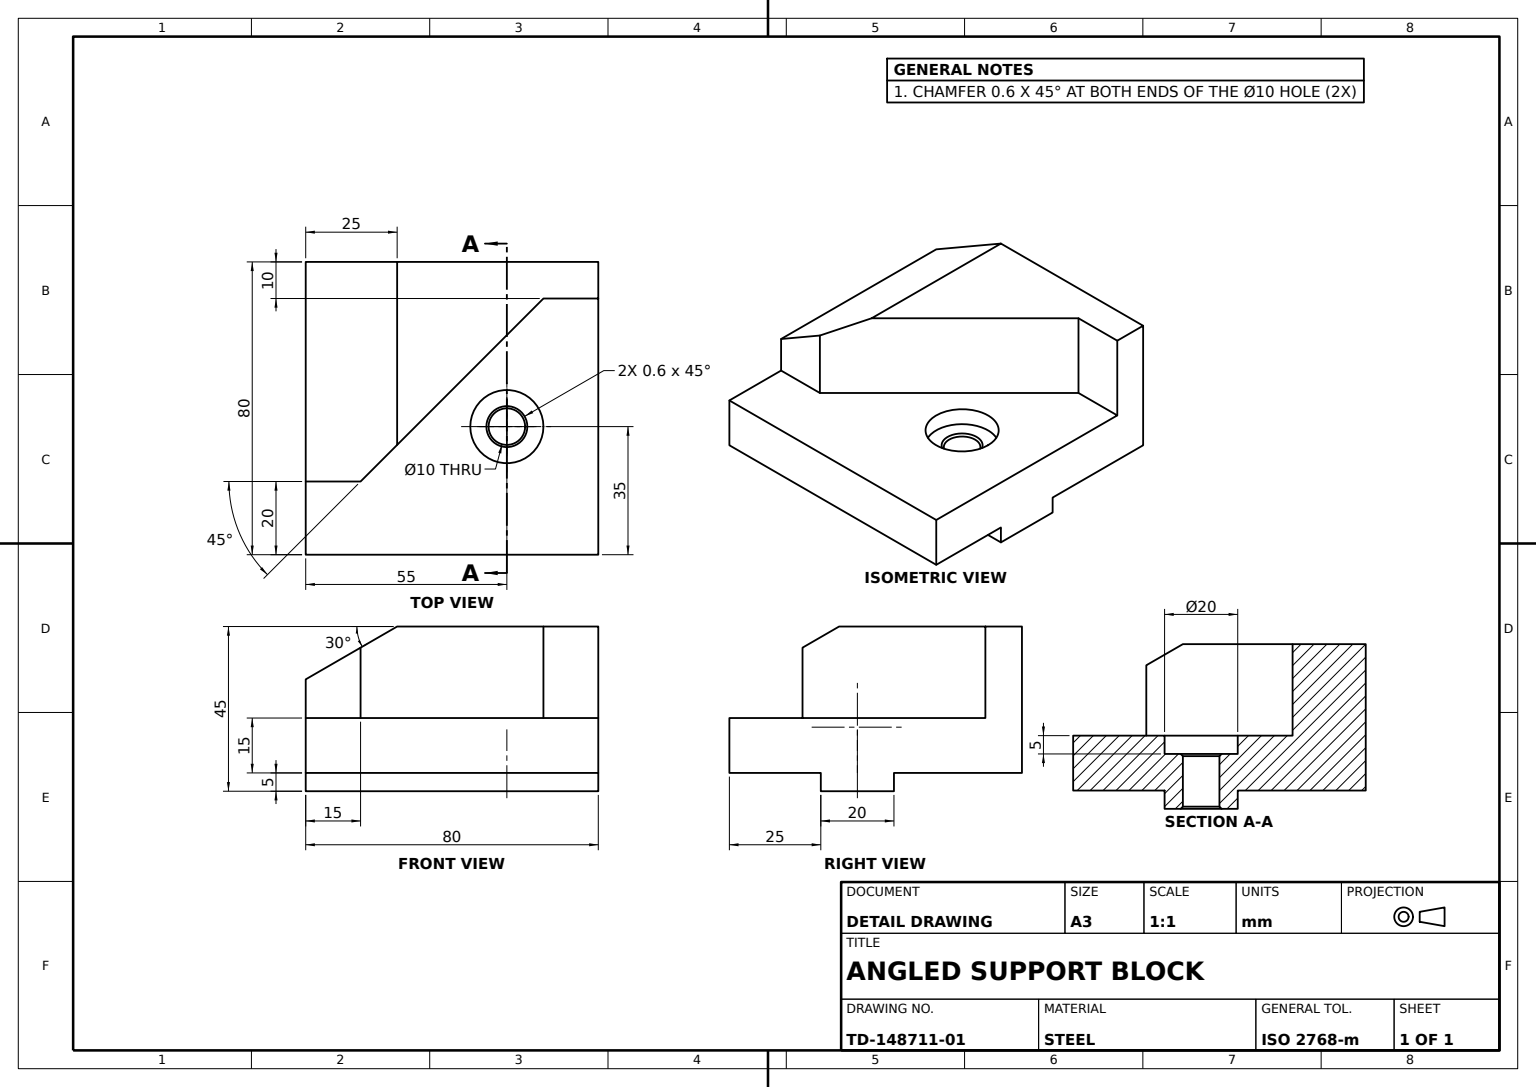
ISO-10303-21;
HEADER;
FILE_DESCRIPTION((''),'2;1');
FILE_NAME('','',(''),(''),'','','');
FILE_SCHEMA(('AUTOMOTIVE_DESIGN'));
ENDSEC;
DATA;
#1=APPLICATION_CONTEXT('');
#2=PRODUCT_CONTEXT('',#1,'mechanical');
#3=PRODUCT('','','',(#2));
#4=PRODUCT_DEFINITION_FORMATION('','',#3);
#5=PRODUCT_DEFINITION_CONTEXT('',#1,'design');
#6=PRODUCT_DEFINITION('','',#4,#5);
#7=PRODUCT_DEFINITION_SHAPE('','',#6);
#8=(LENGTH_UNIT()NAMED_UNIT(*)SI_UNIT(.MILLI.,.METRE.));
#9=(NAMED_UNIT(*)PLANE_ANGLE_UNIT()SI_UNIT($,.RADIAN.));
#10=(NAMED_UNIT(*)SI_UNIT($,.STERADIAN.)SOLID_ANGLE_UNIT());
#11=UNCERTAINTY_MEASURE_WITH_UNIT(LENGTH_MEASURE(0.005),#8,'distance_accuracy_value','');
#12=(GEOMETRIC_REPRESENTATION_CONTEXT(3)GLOBAL_UNCERTAINTY_ASSIGNED_CONTEXT((#11))GLOBAL_UNIT_ASSIGNED_CONTEXT((#8,#9,#10))REPRESENTATION_CONTEXT('',''));
#13=CARTESIAN_POINT('',(-15.,40.,40.));
#14=VERTEX_POINT('',#13);
#15=CARTESIAN_POINT('',(-40.,40.,25.566243));
#16=VERTEX_POINT('',#15);
#17=CARTESIAN_POINT('',(15.424682,40.,57.565699));
#18=DIRECTION('',(-0.866025404,0.,-0.5));
#19=VECTOR('',#18,1000.);
#20=LINE('',#17,#19);
#21=EDGE_CURVE('',#14,#16,#20,.T.);
#22=ORIENTED_EDGE('',*,*,#21,.T.);
#23=CARTESIAN_POINT('',(-40.,-20.,25.566243));
#24=VERTEX_POINT('',#23);
#25=CARTESIAN_POINT('',(-40.,-40.,25.566243));
#26=DIRECTION('',(0.,1.,0.));
#27=VECTOR('',#26,1000.);
#28=LINE('',#25,#27);
#29=EDGE_CURVE('',#24,#16,#28,.T.);
#30=ORIENTED_EDGE('',*,*,#29,.F.);
#31=CARTESIAN_POINT('',(-25.,-20.,34.226497));
#32=VERTEX_POINT('',#31);
#33=CARTESIAN_POINT('',(-22.5,-20.,35.669873));
#34=DIRECTION('',(0.866025404,0.,0.5));
#35=VECTOR('',#34,1000.);
#36=LINE('',#33,#35);
#37=EDGE_CURVE('',#24,#32,#36,.T.);
#38=ORIENTED_EDGE('',*,*,#37,.T.);
#39=CARTESIAN_POINT('',(-15.,-10.,40.));
#40=VERTEX_POINT('',#39);
#41=CARTESIAN_POINT('',(19.285714,24.285714,59.794866));
#42=DIRECTION('',(0.654653671,0.654653671,0.377964473));
#43=VECTOR('',#42,1000.);
#44=LINE('',#41,#43);
#45=EDGE_CURVE('',#32,#40,#44,.T.);
#46=ORIENTED_EDGE('',*,*,#45,.T.);
#47=CARTESIAN_POINT('',(-15.,-40.,40.));
#48=LINE('',#47,#27);
#49=EDGE_CURVE('',#40,#14,#48,.T.);
#50=ORIENTED_EDGE('',*,*,#49,.T.);
#51=EDGE_LOOP('',(#22,#30,#38,#46,#50));
#52=FACE_BOUND('',#51,.T.);
#53=DIRECTION('',(0.5,0.,-0.866025404));
#54=AXIS2_PLACEMENT_3D('',#47,#53,#18);
#55=PLANE('',#54);
#56=ADVANCED_FACE('',(#52),#55,.F.);
#57=CARTESIAN_POINT('',(15.,0.6,-5.));
#58=VERTEX_POINT('',#57);
#59=CARTESIAN_POINT('',(15.,-5.,-5.));
#60=DIRECTION('',(0.,0.,-1.));
#61=AXIS2_PLACEMENT_3D('',#59,#60,#26);
#62=CIRCLE('',#61,5.6);
#63=EDGE_CURVE('',#58,#58,#62,.F.);
#64=ORIENTED_EDGE('',*,*,#63,.T.);
#65=EDGE_LOOP('',(#64));
#66=FACE_BOUND('',#65,.T.);
#67=CARTESIAN_POINT('',(40.,-15.,-5.));
#68=VERTEX_POINT('',#67);
#69=CARTESIAN_POINT('',(-40.,-15.,-5.));
#70=VERTEX_POINT('',#69);
#71=DIRECTION('',(-1.,0.,0.));
#72=VECTOR('',#71,1000.);
#73=LINE('',#67,#72);
#74=EDGE_CURVE('',#68,#70,#73,.T.);
#75=ORIENTED_EDGE('',*,*,#74,.T.);
#76=CARTESIAN_POINT('',(-40.,5.,-5.));
#77=VERTEX_POINT('',#76);
#78=DIRECTION('',(0.,-1.,0.));
#79=VECTOR('',#78,1000.);
#80=LINE('',#76,#79);
#81=EDGE_CURVE('',#77,#70,#80,.T.);
#82=ORIENTED_EDGE('',*,*,#81,.F.);
#83=CARTESIAN_POINT('',(40.,5.,-5.));
#84=VERTEX_POINT('',#83);
#85=LINE('',#83,#72);
#86=EDGE_CURVE('',#84,#77,#85,.T.);
#87=ORIENTED_EDGE('',*,*,#86,.F.);
#88=LINE('',#83,#79);
#89=EDGE_CURVE('',#84,#68,#88,.T.);
#90=ORIENTED_EDGE('',*,*,#89,.T.);
#91=EDGE_LOOP('',(#75,#82,#87,#90));
#92=FACE_BOUND('',#91,.T.);
#93=AXIS2_PLACEMENT_3D('',#83,#60,#26);
#94=PLANE('',#93);
#95=ADVANCED_FACE('',(#66,#92),#94,.T.);
#96=CARTESIAN_POINT('',(40.,30.,40.));
#97=VERTEX_POINT('',#96);
#98=CARTESIAN_POINT('',(25.,30.,40.));
#99=VERTEX_POINT('',#98);
#100=LINE('',#96,#72);
#101=EDGE_CURVE('',#97,#99,#100,.T.);
#102=ORIENTED_EDGE('',*,*,#101,.T.);
#103=CARTESIAN_POINT('',(25.,30.,15.));
#104=VERTEX_POINT('',#103);
#105=VECTOR('',#60,1000.);
#106=LINE('',#98,#105);
#107=EDGE_CURVE('',#99,#104,#106,.T.);
#108=ORIENTED_EDGE('',*,*,#107,.T.);
#109=CARTESIAN_POINT('',(40.,30.,15.));
#110=VERTEX_POINT('',#109);
#111=LINE('',#109,#72);
#112=EDGE_CURVE('',#110,#104,#111,.T.);
#113=ORIENTED_EDGE('',*,*,#112,.F.);
#114=LINE('',#96,#105);
#115=EDGE_CURVE('',#97,#110,#114,.T.);
#116=ORIENTED_EDGE('',*,*,#115,.F.);
#117=EDGE_LOOP('',(#102,#108,#113,#116));
#118=FACE_BOUND('',#117,.T.);
#119=DIRECTION('',(0.,0.,1.));
#120=AXIS2_PLACEMENT_3D('',#96,#26,#119);
#121=PLANE('',#120);
#122=ADVANCED_FACE('',(#118),#121,.F.);
#123=CARTESIAN_POINT('',(-40.,-40.,0.));
#124=VERTEX_POINT('',#123);
#125=CARTESIAN_POINT('',(-40.,-40.,15.));
#126=VERTEX_POINT('',#125);
#127=VECTOR('',#119,1000.);
#128=LINE('',#123,#127);
#129=EDGE_CURVE('',#124,#126,#128,.T.);
#130=ORIENTED_EDGE('',*,*,#129,.F.);
#131=CARTESIAN_POINT('',(40.,-40.,0.));
#132=VERTEX_POINT('',#131);
#133=LINE('',#131,#72);
#134=EDGE_CURVE('',#132,#124,#133,.T.);
#135=ORIENTED_EDGE('',*,*,#134,.F.);
#136=CARTESIAN_POINT('',(40.,-40.,15.));
#137=VERTEX_POINT('',#136);
#138=LINE('',#131,#127);
#139=EDGE_CURVE('',#132,#137,#138,.T.);
#140=ORIENTED_EDGE('',*,*,#139,.T.);
#141=LINE('',#136,#72);
#142=EDGE_CURVE('',#137,#126,#141,.T.);
#143=ORIENTED_EDGE('',*,*,#142,.T.);
#144=EDGE_LOOP('',(#130,#135,#140,#143));
#145=FACE_BOUND('',#144,.T.);
#146=AXIS2_PLACEMENT_3D('',#131,#78,#60);
#147=PLANE('',#146);
#148=ADVANCED_FACE('',(#145),#147,.T.);
#149=CARTESIAN_POINT('',(10.,-5.,-4.4));
#150=VERTEX_POINT('',#149);
#151=CARTESIAN_POINT('',(15.,-5.,-4.4));
#152=AXIS2_PLACEMENT_3D('',#151,#60,#71);
#153=CIRCLE('',#152,5.);
#154=EDGE_CURVE('',#150,#150,#153,.T.);
#155=ORIENTED_EDGE('',*,*,#154,.F.);
#156=EDGE_LOOP('',(#155));
#157=FACE_BOUND('',#156,.T.);
#158=ORIENTED_EDGE('',*,*,#63,.F.);
#159=EDGE_LOOP('',(#158));
#160=FACE_BOUND('',#159,.T.);
#161=CONICAL_SURFACE('',#152,5.,0.785398163);
#162=ADVANCED_FACE('',(#157,#160),#161,.F.);
#163=LINE('',#136,#27);
#164=EDGE_CURVE('',#137,#110,#163,.T.);
#165=ORIENTED_EDGE('',*,*,#164,.F.);
#166=ORIENTED_EDGE('',*,*,#139,.F.);
#167=CARTESIAN_POINT('',(40.,-15.,0.));
#168=VERTEX_POINT('',#167);
#169=CARTESIAN_POINT('',(40.,40.,0.));
#170=LINE('',#169,#79);
#171=EDGE_CURVE('',#168,#132,#170,.T.);
#172=ORIENTED_EDGE('',*,*,#171,.F.);
#173=LINE('',#67,#127);
#174=EDGE_CURVE('',#68,#168,#173,.T.);
#175=ORIENTED_EDGE('',*,*,#174,.F.);
#176=ORIENTED_EDGE('',*,*,#89,.F.);
#177=CARTESIAN_POINT('',(40.,5.,0.));
#178=VERTEX_POINT('',#177);
#179=CARTESIAN_POINT('',(40.,5.,9.745919));
#180=LINE('',#179,#105);
#181=EDGE_CURVE('',#178,#84,#180,.T.);
#182=ORIENTED_EDGE('',*,*,#181,.F.);
#183=VERTEX_POINT('',#169);
#184=EDGE_CURVE('',#183,#178,#170,.T.);
#185=ORIENTED_EDGE('',*,*,#184,.F.);
#186=CARTESIAN_POINT('',(40.,40.,40.));
#187=VERTEX_POINT('',#186);
#188=CARTESIAN_POINT('',(40.,40.,15.));
#189=LINE('',#188,#105);
#190=EDGE_CURVE('',#187,#183,#189,.T.);
#191=ORIENTED_EDGE('',*,*,#190,.F.);
#192=LINE('',#186,#79);
#193=EDGE_CURVE('',#187,#97,#192,.T.);
#194=ORIENTED_EDGE('',*,*,#193,.T.);
#195=ORIENTED_EDGE('',*,*,#115,.T.);
#196=EDGE_LOOP('',(#165,#166,#172,#175,#176,#182,#185,#191,#194,#195));
#197=FACE_BOUND('',#196,.T.);
#198=CARTESIAN_POINT('',(40.,0.,0.));
#199=AXIS2_PLACEMENT_3D('',#198,#71,#119);
#200=PLANE('',#199);
#201=ADVANCED_FACE('',(#197),#200,.F.);
#202=ORIENTED_EDGE('',*,*,#86,.T.);
#203=CARTESIAN_POINT('',(-40.,5.,0.));
#204=VERTEX_POINT('',#203);
#205=CARTESIAN_POINT('',(-40.,5.,9.745919));
#206=LINE('',#205,#105);
#207=EDGE_CURVE('',#204,#77,#206,.T.);
#208=ORIENTED_EDGE('',*,*,#207,.F.);
#209=DIRECTION('',(1.,0.,0.));
#210=VECTOR('',#209,1000.);
#211=LINE('',#177,#210);
#212=EDGE_CURVE('',#204,#178,#211,.T.);
#213=ORIENTED_EDGE('',*,*,#212,.T.);
#214=ORIENTED_EDGE('',*,*,#181,.T.);
#215=EDGE_LOOP('',(#202,#208,#213,#214));
#216=FACE_BOUND('',#215,.T.);
#217=AXIS2_PLACEMENT_3D('',#179,#26,#119);
#218=PLANE('',#217);
#219=ADVANCED_FACE('',(#216),#218,.T.);
#220=CARTESIAN_POINT('',(-25.,-20.,15.));
#221=VERTEX_POINT('',#220);
#222=CARTESIAN_POINT('',(-25.,-20.,40.));
#223=LINE('',#222,#105);
#224=EDGE_CURVE('',#32,#221,#223,.T.);
#225=ORIENTED_EDGE('',*,*,#224,.T.);
#226=CARTESIAN_POINT('',(-2.5,2.5,15.));
#227=DIRECTION('',(0.707106781,0.707106781,0.));
#228=VECTOR('',#227,1000.);
#229=LINE('',#226,#228);
#230=EDGE_CURVE('',#221,#104,#229,.T.);
#231=ORIENTED_EDGE('',*,*,#230,.T.);
#232=ORIENTED_EDGE('',*,*,#107,.F.);
#233=DIRECTION('',(-0.707106781,-0.707106781,0.));
#234=VECTOR('',#233,1000.);
#235=LINE('',#98,#234);
#236=EDGE_CURVE('',#99,#40,#235,.T.);
#237=ORIENTED_EDGE('',*,*,#236,.T.);
#238=ORIENTED_EDGE('',*,*,#45,.F.);
#239=EDGE_LOOP('',(#225,#231,#232,#237,#238));
#240=FACE_BOUND('',#239,.T.);
#241=DIRECTION('',(0.707106781,-0.707106781,0.));
#242=AXIS2_PLACEMENT_3D('',#98,#241,#227);
#243=PLANE('',#242);
#244=ADVANCED_FACE('',(#240),#243,.T.);
#245=ORIENTED_EDGE('',*,*,#74,.F.);
#246=ORIENTED_EDGE('',*,*,#174,.T.);
#247=CARTESIAN_POINT('',(-40.,-15.,0.));
#248=VERTEX_POINT('',#247);
#249=LINE('',#167,#72);
#250=EDGE_CURVE('',#168,#248,#249,.T.);
#251=ORIENTED_EDGE('',*,*,#250,.T.);
#252=LINE('',#69,#127);
#253=EDGE_CURVE('',#70,#248,#252,.T.);
#254=ORIENTED_EDGE('',*,*,#253,.F.);
#255=EDGE_LOOP('',(#245,#246,#251,#254));
#256=FACE_BOUND('',#255,.T.);
#257=AXIS2_PLACEMENT_3D('',#67,#78,#60);
#258=PLANE('',#257);
#259=ADVANCED_FACE('',(#256),#258,.T.);
#260=CARTESIAN_POINT('',(25.,-5.,15.));
#261=VERTEX_POINT('',#260);
#262=CARTESIAN_POINT('',(15.,-5.,15.));
#263=AXIS2_PLACEMENT_3D('',#262,#119,#209);
#264=CIRCLE('',#263,10.);
#265=EDGE_CURVE('',#261,#261,#264,.F.);
#266=ORIENTED_EDGE('',*,*,#265,.T.);
#267=EDGE_LOOP('',(#266));
#268=FACE_BOUND('',#267,.T.);
#269=ORIENTED_EDGE('',*,*,#230,.F.);
#270=CARTESIAN_POINT('',(-40.,-20.,15.));
#271=VERTEX_POINT('',#270);
#272=CARTESIAN_POINT('',(40.,-20.,15.));
#273=LINE('',#272,#210);
#274=EDGE_CURVE('',#271,#221,#273,.T.);
#275=ORIENTED_EDGE('',*,*,#274,.F.);
#276=LINE('',#125,#27);
#277=EDGE_CURVE('',#126,#271,#276,.T.);
#278=ORIENTED_EDGE('',*,*,#277,.F.);
#279=ORIENTED_EDGE('',*,*,#142,.F.);
#280=ORIENTED_EDGE('',*,*,#164,.T.);
#281=ORIENTED_EDGE('',*,*,#112,.T.);
#282=EDGE_LOOP('',(#269,#275,#278,#279,#280,#281));
#283=FACE_BOUND('',#282,.T.);
#284=AXIS2_PLACEMENT_3D('',#136,#119,#209);
#285=PLANE('',#284);
#286=ADVANCED_FACE('',(#268,#283),#285,.T.);
#287=CARTESIAN_POINT('',(20.,-5.,9.4));
#288=VERTEX_POINT('',#287);
#289=CARTESIAN_POINT('',(15.,-5.,9.4));
#290=AXIS2_PLACEMENT_3D('',#289,#119,#209);
#291=CIRCLE('',#290,5.);
#292=EDGE_CURVE('',#288,#288,#291,.T.);
#293=ORIENTED_EDGE('',*,*,#292,.T.);
#294=EDGE_LOOP('',(#293));
#295=FACE_BOUND('',#294,.T.);
#296=ORIENTED_EDGE('',*,*,#154,.T.);
#297=EDGE_LOOP('',(#296));
#298=FACE_BOUND('',#297,.T.);
#299=CARTESIAN_POINT('',(15.,-5.,10.));
#300=AXIS2_PLACEMENT_3D('',#299,#60,#71);
#301=CYLINDRICAL_SURFACE('',#300,5.);
#302=ADVANCED_FACE('',(#295,#298),#301,.F.);
#303=CARTESIAN_POINT('',(25.,-5.,10.));
#304=VERTEX_POINT('',#303);
#305=AXIS2_PLACEMENT_3D('',#299,#119,#209);
#306=CIRCLE('',#305,10.);
#307=EDGE_CURVE('',#304,#304,#306,.F.);
#308=ORIENTED_EDGE('',*,*,#307,.T.);
#309=EDGE_LOOP('',(#308));
#310=FACE_BOUND('',#309,.T.);
#311=ORIENTED_EDGE('',*,*,#265,.F.);
#312=EDGE_LOOP('',(#311));
#313=FACE_BOUND('',#312,.T.);
#314=CARTESIAN_POINT('',(15.,-5.,26.5));
#315=AXIS2_PLACEMENT_3D('',#314,#60,#71);
#316=CYLINDRICAL_SURFACE('',#315,10.);
#317=ADVANCED_FACE('',(#310,#313),#316,.F.);
#318=ORIENTED_EDGE('',*,*,#292,.F.);
#319=EDGE_LOOP('',(#318));
#320=FACE_BOUND('',#319,.T.);
#321=CARTESIAN_POINT('',(20.6,-5.,10.));
#322=VERTEX_POINT('',#321);
#323=CIRCLE('',#305,5.6);
#324=EDGE_CURVE('',#322,#322,#323,.F.);
#325=ORIENTED_EDGE('',*,*,#324,.F.);
#326=EDGE_LOOP('',(#325));
#327=FACE_BOUND('',#326,.T.);
#328=CONICAL_SURFACE('',#305,5.6,0.785398163);
#329=ADVANCED_FACE('',(#320,#327),#328,.F.);
#330=CARTESIAN_POINT('',(-40.,40.,0.));
#331=VERTEX_POINT('',#330);
#332=CARTESIAN_POINT('',(-40.,40.,15.));
#333=LINE('',#332,#105);
#334=EDGE_CURVE('',#16,#331,#333,.T.);
#335=ORIENTED_EDGE('',*,*,#334,.F.);
#336=ORIENTED_EDGE('',*,*,#21,.F.);
#337=LINE('',#186,#72);
#338=EDGE_CURVE('',#187,#14,#337,.T.);
#339=ORIENTED_EDGE('',*,*,#338,.F.);
#340=ORIENTED_EDGE('',*,*,#190,.T.);
#341=LINE('',#169,#72);
#342=EDGE_CURVE('',#183,#331,#341,.T.);
#343=ORIENTED_EDGE('',*,*,#342,.T.);
#344=EDGE_LOOP('',(#335,#336,#339,#340,#343));
#345=FACE_BOUND('',#344,.T.);
#346=AXIS2_PLACEMENT_3D('',#188,#26,#119);
#347=PLANE('',#346);
#348=ADVANCED_FACE('',(#345),#347,.T.);
#349=ORIENTED_EDGE('',*,*,#253,.T.);
#350=LINE('',#330,#79);
#351=EDGE_CURVE('',#248,#124,#350,.T.);
#352=ORIENTED_EDGE('',*,*,#351,.T.);
#353=ORIENTED_EDGE('',*,*,#129,.T.);
#354=ORIENTED_EDGE('',*,*,#277,.T.);
#355=CARTESIAN_POINT('',(-40.,-20.,40.));
#356=LINE('',#355,#105);
#357=EDGE_CURVE('',#24,#271,#356,.T.);
#358=ORIENTED_EDGE('',*,*,#357,.F.);
#359=ORIENTED_EDGE('',*,*,#29,.T.);
#360=ORIENTED_EDGE('',*,*,#334,.T.);
#361=EDGE_CURVE('',#331,#204,#350,.T.);
#362=ORIENTED_EDGE('',*,*,#361,.T.);
#363=ORIENTED_EDGE('',*,*,#207,.T.);
#364=ORIENTED_EDGE('',*,*,#81,.T.);
#365=EDGE_LOOP('',(#349,#352,#353,#354,#358,#359,#360,#362,#363,#364));
#366=FACE_BOUND('',#365,.T.);
#367=CARTESIAN_POINT('',(-40.,0.,0.));
#368=AXIS2_PLACEMENT_3D('',#367,#71,#119);
#369=PLANE('',#368);
#370=ADVANCED_FACE('',(#366),#369,.T.);
#371=ORIENTED_EDGE('',*,*,#274,.T.);
#372=ORIENTED_EDGE('',*,*,#224,.F.);
#373=ORIENTED_EDGE('',*,*,#37,.F.);
#374=ORIENTED_EDGE('',*,*,#357,.T.);
#375=EDGE_LOOP('',(#371,#372,#373,#374));
#376=FACE_BOUND('',#375,.T.);
#377=AXIS2_PLACEMENT_3D('',#222,#78,#209);
#378=PLANE('',#377);
#379=ADVANCED_FACE('',(#376),#378,.T.);
#380=ORIENTED_EDGE('',*,*,#361,.F.);
#381=ORIENTED_EDGE('',*,*,#342,.F.);
#382=ORIENTED_EDGE('',*,*,#184,.T.);
#383=ORIENTED_EDGE('',*,*,#212,.F.);
#384=EDGE_LOOP('',(#380,#381,#382,#383));
#385=FACE_BOUND('',#384,.T.);
#386=AXIS2_PLACEMENT_3D('',#169,#60,#26);
#387=PLANE('',#386);
#388=ADVANCED_FACE('',(#385),#387,.T.);
#389=ORIENTED_EDGE('',*,*,#351,.F.);
#390=ORIENTED_EDGE('',*,*,#250,.F.);
#391=ORIENTED_EDGE('',*,*,#171,.T.);
#392=ORIENTED_EDGE('',*,*,#134,.T.);
#393=EDGE_LOOP('',(#389,#390,#391,#392));
#394=FACE_BOUND('',#393,.T.);
#395=ADVANCED_FACE('',(#394),#387,.T.);
#396=ORIENTED_EDGE('',*,*,#324,.T.);
#397=EDGE_LOOP('',(#396));
#398=FACE_BOUND('',#397,.T.);
#399=ORIENTED_EDGE('',*,*,#307,.F.);
#400=EDGE_LOOP('',(#399));
#401=FACE_BOUND('',#400,.T.);
#402=PLANE('',#305);
#403=ADVANCED_FACE('',(#398,#401),#402,.T.);
#404=ORIENTED_EDGE('',*,*,#236,.F.);
#405=ORIENTED_EDGE('',*,*,#101,.F.);
#406=ORIENTED_EDGE('',*,*,#193,.F.);
#407=ORIENTED_EDGE('',*,*,#338,.T.);
#408=ORIENTED_EDGE('',*,*,#49,.F.);
#409=EDGE_LOOP('',(#404,#405,#406,#407,#408));
#410=FACE_BOUND('',#409,.T.);
#411=AXIS2_PLACEMENT_3D('',#186,#60,#26);
#412=PLANE('',#411);
#413=ADVANCED_FACE('',(#410),#412,.F.);
#414=CLOSED_SHELL('',(#56,#95,#122,#148,#162,#201,#219,#244,#259,#286,#302,#317,#329,#348,#370,#379,#388,#395,#403,#413));
#415=MANIFOLD_SOLID_BREP('',#414);
#416=ADVANCED_BREP_SHAPE_REPRESENTATION('',(#415),#12);
#417=SHAPE_DEFINITION_REPRESENTATION(#7,#416);
ENDSEC;
END-ISO-10303-21;
